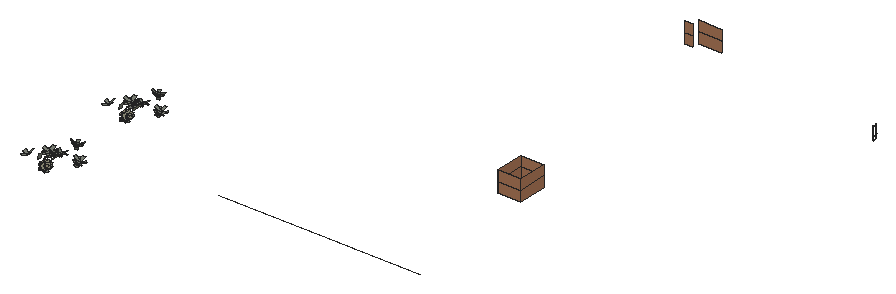
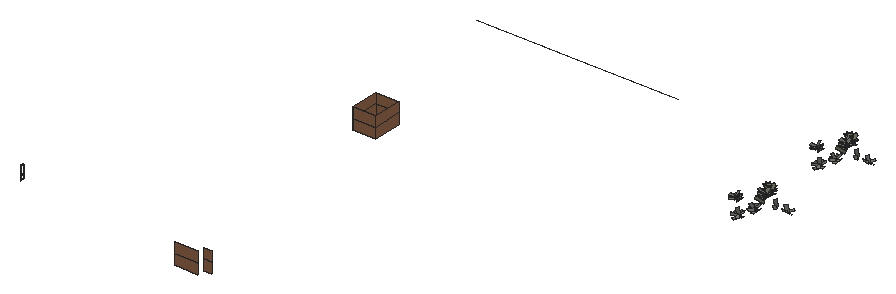
# SketchUp Ruby script. Lengths in inches.
U = 1.inch
M = Sketchup.active_model
def pt(a) = Geom::Point3d.new(a.map { |v| v * U })
def face(e, loops, mat)
  f = e.add_face(loops[0].map { |a| pt(a) })
  loops[1..].each { |l| e.add_face(l.map { |a| pt(a) }).erase! }
  f.material = f.back_material = mat if mat
  f
end
# faces: each face lists its corners as indices into pts; further lists are holes
def faces(e, pts, list, mat = nil) = list.each { |f| face(e, (f[0].is_a?(Array) ? f : [f]).map { |l| l.map { |i| pts[i] } }, mat) }
# xy, xz, yz: faces in a plane at the given z, y or x. An outline is a flat list of corners, or four numbers for a rectangle; further outlines are holes
def ring(l) = l.size == 4 ? [[l[0], l[1]], [l[2], l[1]], [l[2], l[3]], [l[0], l[3]]] : l.each_slice(2).to_a
def flat(e, list, mat, &to3) = list.each { |f| face(e, (f[0].is_a?(Array) ? f : [f]).map { |l| ring(l).map { |u, v| to3.(u, v) } }, mat) }
def xy(e, z, list, mat = nil) = flat(e, list, mat) { |x, y| [x, y, z] }
def xz(e, y, list, mat = nil) = flat(e, list, mat) { |x, z| [x, y, z] }
def yz(e, x, list, mat = nil) = flat(e, list, mat) { |y, z| [x, y, z] }
def lines(e, pts, list) = list.each { |a, b| e.add_line(pt(pts[a]), pt(pts[b])) }
# prism: a flat outline (further loops are holes) pulled along v
def prism(e, loops, v, mat = nil)
  f = face(e, loops, mat); d = Geom::Vector3d.new(v.map { |x| x * U })
  f.pushpull(f.normal.samedirection?(d) ? d.length : -d.length)
end
def box(e, o, s, mat = nil) = prism(e, [[o, [o[0] + s[0], o[1], o[2]], [o[0] + s[0], o[1] + s[1], o[2]], [o[0], o[1] + s[1], o[2]]]], [0, 0, s[2]], mat)
def at(x, y, z, deg = 0) = Geom::Transformation.translation(pt([x, y, z])) * Geom::Transformation.rotation(ORIGIN, Z_AXIS, deg.degrees)
def axes(o, x, y, z) = Geom::Transformation.new([*x, 0, *y, 0, *z, 0, *pt(o).to_a, 1])
def part(name) = M.definitions.add(name)
# library, detail: a bought-in or finely detailed component or shape, given as its bounding box
def library(name, o, s) = part(name).tap { |d| box(d.entities, o, s) }
def detail(e, o, s) = box(e.add_group.entities, o, s)
def put(e, d, t, mat = nil) = e.add_instance(d, t).tap { |i| i.material = mat if mat }
def group(e, t, mat = nil) = e.add_group.tap { |g| g.transformation = t; g.material = mat if mat }.entities
root = M.entities
M.materials.add("Material \#1").color = [140, 140, 140]
M.materials.add("[Tile Ceramic Multi]").color = [165, 115, 84]
M.materials.add("viburnumblaasdfas0df1w06d").color = [98, 102, 84]
M.materials.add("viburnumbladsadfasdfad0w122").color = [125, 129, 119]
M.materials.add("viburnumbloem1asdfas0d1fas0d616w").color = [137, 130, 109]
M.materials.add("viburnumbloem2asdfas01vxc5016").color = [175, 173, 148]
c1 = part("Component\#315")
p = [[0.25,0,0],[2.05,0.01,0.35],[1.81,4.2,1.66],[0,4.19,1.3125]]
faces(c1.entities,p,[[0,1,2,3]],"viburnumbladsadfasdfad0w122")
c2 = part("viburnumblad2")
put(c2.entities,c1,axes([-19.23,-4.49,-32.18],[83.35428,0,0],[0,79.38502,0],[0,0,83.35428]))
c3 = part("Component\#314")
p = [[0.14,0,0],[2.58,0.05,0.25],[2.44,5.11,2.64],[0,5.05,2.39]]
faces(c3.entities,p,[[0,1,2,3]],"viburnumblaasdfas0df1w06d")
c4 = part("viburnumblad1\#2")
put(c4.entities,c3,axes([-37.25,6.23,19.31],[75.98784,0,0],[0,65.50676,0],[0,0,75.98784]))
c5 = part("Component\#334")
p = [[0.16,3.84,5.17],[0,4.97,1.27],[3.78,1.125,0],[3.9375,0,3.9]]
faces(c5.entities,p,[[0,1,2,3]],"viburnumbloem2asdfas01vxc5016")
c6 = part("Component\#335")
p = [[1.35,5.21,5.35],[1.19,6.33,1.45],[0,1.125,0],[0.16,0,3.9]]
faces(c6.entities,p,[[0,1,2,3]],"viburnumbloem2asdfas01vxc5016")
c7 = part("Component\#333")
p = [[6.15,4.98,1.43],[0.18,5.1,1.71],[0,0.13,0.29],[5.97,0,0]]
faces(c7.entities,p,[[0,1,2,3]],"viburnumbloem1asdfas0d1fas0d616w")
c8 = part("Component\#336")
p = [[6.03,1.45,4.43],[5.85,2.68,0.17],[0,1.22,0],[0.18,0,4.25]]
faces(c8.entities,p,[[0,1,2,3]],"viburnumbloem2asdfas01vxc5016")
xz(root,340.216,[[1457.075,40,1474.638,48],[1457.075,48,1474.638,56]],"[Tile Ceramic Multi]")
xz(root,362.068,[[1457.075,40,1474.638,48],[1457.075,48,1474.638,56]],"[Tile Ceramic Multi]")
xz(root,529.3125,[[1590.723,42.477,1590.719,42.483,1590.583,42.689],[1590.719,42.483,1590.713,42.489,1590.583,42.689],[1590.713,42.489,1590.648,42.548,1590.583,42.689],[1590.713,42.489,1590.707,42.494,1590.648,42.548],[1590.707,42.494,1590.675,42.519,1590.648,42.548],
  [1590.648,42.548,1590.606,42.614,1590.583,42.689],[1590.648,42.548,1590.625,42.58,1590.606,42.614],[1590.686,42.562,1590.583,42.689,1590.651,42.612],[1590.651,42.612,1590.583,42.689,1590.628,42.668],[1590.606,42.614,1590.592,42.65,1590.583,42.689],
  [1590.628,42.668,1590.583,42.689,1590.62,42.729],[1590.583,42.689,1590.58,42.729,1590.589,42.798],[1590.583,42.689,1590.589,42.798,1590.655,42.918],[1590.583,42.689,1590.628,42.79,1590.62,42.729],[1590.583,42.689,1590.655,42.918,1590.628,42.79],
  [1590.628,42.79,1590.655,42.918,1590.651,42.846],[1590.589,42.798,1590.615,42.862,1590.655,42.918],[1590.651,42.846,1590.655,42.918,1590.686,42.896],[1590.686,42.896,1590.655,42.918,1590.733,42.9375],[1590.655,42.918,1590.708,42.965,1590.771,43.001],
  [1590.655,42.918,1590.788,42.969,1590.733,42.9375]],"Material \#1")
xz(root,529.347,[[1590.251,39.557,1590.17,39.659,1590.263,39.566],[1590.743,39.559,1590.698,39.58,1590.71,39.589],[1590.263,39.566,1590.17,39.659,1590.183,39.666],[1590.698,39.58,1590.669,39.616,1590.71,39.589],[1590.71,39.589,1590.669,39.616,1590.682,39.623],
  [1590.669,39.616,1590.648,39.657,1590.682,39.623],[1590.682,39.623,1590.648,39.657,1590.662,39.661],[1590.648,39.657,1590.634,39.701,1590.662,39.661],[1590.17,39.659,1590.1,39.787,1590.183,39.666],[1590.662,39.661,1590.634,39.701,1590.649,39.703],
  [1590.183,39.666,1590.1,39.787,1590.115,39.792],[1590.634,39.701,1590.63,39.742,1590.649,39.703],[1590.649,39.703,1590.63,39.742,1590.645,39.742],[1590.63,39.742,1590.634,39.793,1590.645,39.742],[1590.645,39.742,1590.634,39.793,1590.649,39.791],
  [1590.1,39.787,1590.06,39.918,1590.115,39.792],[1590.649,39.791,1590.634,39.793,1590.648,39.837],[1590.649,39.791,1590.648,39.837,1590.662,39.832],[1590.115,39.792,1590.06,39.918,1590.075,39.921],[1590.662,39.832,1590.648,39.837,1590.669,39.877],
  [1590.662,39.832,1590.669,39.877,1590.682,39.871],[1590.682,39.871,1590.669,39.877,1590.698,39.913],[1590.682,39.871,1590.698,39.913,1590.71,39.905],[1590.71,39.905,1590.698,39.913,1590.733,39.945],[1590.06,39.918,1590.045,40.063,1590.075,39.921],
  [1590.075,39.921,1590.045,40.063,1590.06,40.064],[1590.045,40.063,1590.045,48.955,1590.06,40.064],[1590.06,40.064,1590.045,48.955,1590.06,48.955],[1590.045,48.955,1590.06,49.1,1590.06,48.955],[1590.06,48.955,1590.06,49.1,1590.075,49.098],
  [1590.743,49.084,1590.698,49.105,1590.71,49.114],[1590.075,49.098,1590.06,49.1,1590.1,49.232],[1590.075,49.098,1590.1,49.232,1590.115,49.227],[1590.698,49.105,1590.669,49.141,1590.71,49.114],[1590.71,49.114,1590.669,49.141,1590.682,49.148],
  [1590.669,49.141,1590.648,49.182,1590.682,49.148],[1590.682,49.148,1590.648,49.182,1590.662,49.186],[1590.648,49.182,1590.634,49.226,1590.662,49.186],[1590.662,49.186,1590.634,49.226,1590.649,49.228],[1590.634,49.226,1590.63,49.284,1590.649,49.228],
  [1590.115,49.227,1590.1,49.232,1590.165,49.353],[1590.115,49.227,1590.165,49.353,1590.178,49.346],[1590.649,49.228,1590.63,49.284,1590.645,49.284],[1590.63,49.284,1590.634,49.318,1590.645,49.284],[1590.645,49.284,1590.634,49.318,1590.649,49.316],
  [1590.649,49.316,1590.634,49.318,1590.648,49.362],[1590.649,49.316,1590.648,49.362,1590.662,49.357],[1590.178,49.346,1590.165,49.353,1590.255,49.465],[1590.178,49.346,1590.255,49.465,1590.267,49.457],[1590.662,49.357,1590.648,49.362,1590.669,49.402],
  [1590.662,49.357,1590.669,49.402,1590.682,49.396],[1590.682,49.396,1590.669,49.402,1590.698,49.438],[1590.682,49.396,1590.698,49.438,1590.71,49.43],[1590.71,49.43,1590.698,49.438,1590.733,49.47],[1590.267,49.457,1590.255,49.465,1590.357,49.556],
  [1590.267,49.457,1590.357,49.556,1590.367,49.545],[1590.367,49.545,1590.357,49.556,1590.479,49.632],[1590.367,49.545,1590.479,49.632,1590.487,49.621],[1590.487,49.621,1590.479,49.632,1590.615,49.69],[1590.487,49.621,1590.615,49.69,1590.62,49.677],
  [1590.62,49.677,1590.615,49.69,1590.763,49.726],[1590.62,49.677,1590.763,49.726,1590.766,49.713]],"Material \#1")
xz(root,529.66,[[1590.723,42.477,1590.583,42.689,1590.719,42.483],[1590.723,42.477,1590.651,42.612,1590.583,42.689],[1590.723,42.477,1590.686,42.562,1590.651,42.612],[1590.719,42.483,1590.583,42.689,1590.713,42.489],[1590.713,42.489,1590.583,42.689,1590.648,42.548],
  [1590.713,42.489,1590.648,42.548,1590.707,42.494],[1590.707,42.494,1590.648,42.548,1590.675,42.519],[1590.648,42.548,1590.583,42.689,1590.606,42.614],[1590.648,42.548,1590.606,42.614,1590.625,42.58],[1590.651,42.612,1590.628,42.668,1590.583,42.689],
  [1590.606,42.614,1590.583,42.689,1590.592,42.65],[1590.628,42.668,1590.62,42.729,1590.583,42.689],[1590.583,42.689,1590.589,42.798,1590.58,42.729],[1590.583,42.689,1590.62,42.729,1590.628,42.79],[1590.583,42.689,1590.628,42.79,1590.651,42.846],
  [1590.583,42.689,1590.651,42.846,1590.655,42.918],[1590.583,42.689,1590.655,42.918,1590.589,42.798],[1590.589,42.798,1590.655,42.918,1590.615,42.862],[1590.651,42.846,1590.686,42.896,1590.655,42.918],[1590.686,42.896,1590.733,42.9375,1590.655,42.918],
  [1590.655,42.918,1590.771,43.001,1590.708,42.965]],"Material \#1")
xz(root,531.048,[[1590.723,42.477,1590.583,42.689,1590.651,42.612],[1590.723,42.477,1590.719,42.483,1590.583,42.689],[1590.723,42.477,1590.651,42.612,1590.686,42.562],[1590.719,42.483,1590.713,42.489,1590.583,42.689],[1590.713,42.489,1590.648,42.548,1590.583,42.689],
  [1590.713,42.489,1590.707,42.494,1590.648,42.548],[1590.707,42.494,1590.675,42.519,1590.648,42.548],[1590.648,42.548,1590.606,42.614,1590.583,42.689],[1590.648,42.548,1590.625,42.58,1590.606,42.614],[1590.651,42.612,1590.583,42.689,1590.628,42.668],
  [1590.606,42.614,1590.592,42.65,1590.583,42.689],[1590.628,42.668,1590.583,42.689,1590.62,42.729],[1590.583,42.689,1590.58,42.729,1590.589,42.798],[1590.583,42.689,1590.589,42.798,1590.655,42.918],[1590.583,42.689,1590.628,42.79,1590.62,42.729],
  [1590.583,42.689,1590.651,42.846,1590.628,42.79],[1590.583,42.689,1590.655,42.918,1590.651,42.846],[1590.589,42.798,1590.615,42.862,1590.655,42.918],[1590.651,42.846,1590.655,42.918,1590.686,42.896],[1590.686,42.896,1590.655,42.918,1590.733,42.9375],
  [1590.655,42.918,1590.708,42.965,1590.771,43.001]],"Material \#1")
xz(root,531.361,[[1590.251,39.557,1590.263,39.566,1590.17,39.659],[1590.263,39.566,1590.183,39.666,1590.17,39.659],[1590.698,39.58,1590.71,39.589,1590.669,39.616],[1590.71,39.589,1590.682,39.623,1590.669,39.616],[1590.669,39.616,1590.682,39.623,1590.648,39.657],
  [1590.682,39.623,1590.662,39.661,1590.648,39.657],[1590.648,39.657,1590.662,39.661,1590.634,39.701],[1590.17,39.659,1590.183,39.666,1590.1,39.787],[1590.662,39.661,1590.649,39.703,1590.634,39.701],[1590.183,39.666,1590.115,39.792,1590.1,39.787],
  [1590.634,39.701,1590.649,39.703,1590.63,39.742],[1590.649,39.703,1590.645,39.742,1590.63,39.742],[1590.63,39.742,1590.645,39.742,1590.634,39.793],[1590.645,39.742,1590.649,39.791,1590.634,39.793],[1590.1,39.787,1590.115,39.792,1590.06,39.918],
  [1590.649,39.791,1590.648,39.837,1590.634,39.793],[1590.649,39.791,1590.662,39.832,1590.648,39.837],[1590.115,39.792,1590.075,39.921,1590.06,39.918],[1590.662,39.832,1590.669,39.877,1590.648,39.837],[1590.662,39.832,1590.682,39.871,1590.669,39.877],
  [1590.682,39.871,1590.698,39.913,1590.669,39.877],[1590.682,39.871,1590.71,39.905,1590.698,39.913],[1590.71,39.905,1590.733,39.945,1590.698,39.913],[1590.06,39.918,1590.075,39.921,1590.045,40.063],[1590.075,39.921,1590.06,40.064,1590.045,40.063],
  [1590.045,40.063,1590.06,40.064,1590.045,48.955],[1590.06,40.064,1590.06,48.955,1590.045,48.955],[1590.045,48.955,1590.06,48.955,1590.06,49.1],[1590.06,48.955,1590.075,49.098,1590.06,49.1],[1590.075,49.098,1590.1,49.232,1590.06,49.1],
  [1590.075,49.098,1590.115,49.227,1590.1,49.232],[1590.698,49.105,1590.71,49.114,1590.669,49.141],[1590.71,49.114,1590.682,49.148,1590.669,49.141],[1590.669,49.141,1590.682,49.148,1590.648,49.182],[1590.682,49.148,1590.662,49.186,1590.648,49.182],
  [1590.648,49.182,1590.662,49.186,1590.634,49.226],[1590.662,49.186,1590.649,49.228,1590.634,49.226],[1590.634,49.226,1590.649,49.228,1590.63,49.284],[1590.115,49.227,1590.165,49.353,1590.1,49.232],[1590.115,49.227,1590.178,49.346,1590.165,49.353],
  [1590.649,49.228,1590.645,49.284,1590.63,49.284],[1590.63,49.284,1590.645,49.284,1590.634,49.318],[1590.645,49.284,1590.649,49.316,1590.634,49.318],[1590.649,49.316,1590.648,49.362,1590.634,49.318],[1590.649,49.316,1590.662,49.357,1590.648,49.362],
  [1590.178,49.346,1590.255,49.465,1590.165,49.353],[1590.178,49.346,1590.267,49.457,1590.255,49.465],[1590.662,49.357,1590.669,49.402,1590.648,49.362],[1590.662,49.357,1590.682,49.396,1590.669,49.402],[1590.682,49.396,1590.698,49.438,1590.669,49.402],
  [1590.682,49.396,1590.71,49.43,1590.698,49.438],[1590.71,49.43,1590.733,49.47,1590.698,49.438],[1590.267,49.457,1590.357,49.556,1590.255,49.465],[1590.267,49.457,1590.367,49.545,1590.357,49.556],[1590.367,49.545,1590.479,49.632,1590.357,49.556],
  [1590.367,49.545,1590.487,49.621,1590.479,49.632],[1590.487,49.621,1590.615,49.69,1590.479,49.632],[1590.487,49.621,1590.62,49.677,1590.615,49.69],[1590.62,49.677,1590.763,49.726,1590.615,49.69],[1590.62,49.677,1590.766,49.713,1590.763,49.726]],"Material \#1")
xz(root,531.396,[[1590.723,42.477,1590.583,42.689,1590.719,42.483],[1590.719,42.483,1590.583,42.689,1590.713,42.489],[1590.713,42.489,1590.583,42.689,1590.648,42.548],[1590.713,42.489,1590.648,42.548,1590.707,42.494],[1590.707,42.494,1590.648,42.548,1590.675,42.519],
  [1590.648,42.548,1590.583,42.689,1590.606,42.614],[1590.648,42.548,1590.606,42.614,1590.625,42.58],[1590.686,42.562,1590.651,42.612,1590.583,42.689],[1590.651,42.612,1590.628,42.668,1590.583,42.689],[1590.606,42.614,1590.583,42.689,1590.592,42.65],
  [1590.628,42.668,1590.62,42.729,1590.583,42.689],[1590.583,42.689,1590.589,42.798,1590.58,42.729],[1590.583,42.689,1590.62,42.729,1590.628,42.79],[1590.583,42.689,1590.628,42.79,1590.655,42.918],[1590.583,42.689,1590.655,42.918,1590.589,42.798],
  [1590.628,42.79,1590.651,42.846,1590.655,42.918],[1590.589,42.798,1590.655,42.918,1590.615,42.862],[1590.651,42.846,1590.686,42.896,1590.655,42.918],[1590.686,42.896,1590.733,42.9375,1590.655,42.918],[1590.655,42.918,1590.771,43.001,1590.708,42.965]],"Material \#1")
xz(root,549.6875,[[1431.3125,40,1437.219,48],[1431.3125,48,1437.219,56]],"[Tile Ceramic Multi]")
xz(root,555,[[1437.219,40,1454.9375,48],[1437.219,48,1454.9375,56]],"[Tile Ceramic Multi]")
yz(root,1457.075,[[340.216,40,362.068,48],[340.216,48,362.068,56]],"[Tile Ceramic Multi]")
yz(root,1474.638,[[340.216,40,362.068,48],[340.216,48,362.068,56]],"[Tile Ceramic Multi]")
p = [[1491.419,223.9375,48],[1338.625,223.9375,48]]
lines(root,p,[[0,1]])
put(root,c2,axes([1210.86,278.68,40.57],[0.00639,0.01034,0.00318],[-0.01046,0.00683,-0.00122],[-0.00247,-0.00201,0.01151]))
put(root,c2,axes([1210.86,201.8,40.57],[0.00639,0.01034,0.00318],[-0.01046,0.00683,-0.00122],[-0.00247,-0.00201,0.01151]))
put(root,c2,axes([1212.37,278.7,41.07],[-0.01008,0.00703,-0.00261],[-0.00679,-0.01041,-0.00178],[-0.00292,0.0001,0.01158]))
put(root,c2,axes([1212.37,201.82,41.07],[-0.01008,0.00703,-0.00261],[-0.00679,-0.01041,-0.00178],[-0.00292,0.0001,0.01158]))
put(root,c2,axes([1210.79,280.26,40.71],[0.01008,-0.00703,0.00261],[0.00588,0.01012,0.00453],[-0.00448,-0.00242,0.01081]))
put(root,c2,axes([1210.79,203.375,40.71],[0.01008,-0.00703,0.00261],[0.00588,0.01012,0.00453],[-0.00448,-0.00242,0.01081]))
put(root,c2,axes([1212.29,280.28,41.21],[-0.00639,-0.01034,-0.00318],[0.00955,-0.00712,0.00396],[-0.00493,-0.0003,0.01087]))
put(root,c2,axes([1212.29,203.4,41.21],[-0.00639,-0.01034,-0.00318],[0.00955,-0.00712,0.00396],[-0.00493,-0.0003,0.01087]))
put(root,c2,axes([1218.84,279.94,40.32],[0.00996,-0.00362,0.00815],[0.00104,0.0126,0.00432],[-0.00886,-0.00258,0.00967]))
put(root,c2,axes([1218.84,203.0625,40.32],[0.00996,-0.00362,0.00815],[0.00104,0.0126,0.00432],[-0.00886,-0.00258,0.00967]))
put(root,c2,axes([1220.02,280.5,41.38],[-0.00212,-0.01282,-0.00311],[0.00883,-0.00372,0.00932],[-0.00981,-0.00058,0.00906]))
put(root,c2,axes([1220.02,203.62,41.38],[-0.00212,-0.01282,-0.00311],[0.00883,-0.00372,0.00932],[-0.00981,-0.00058,0.00906]))
put(root,c2,axes([1227.75,278.98,47.84],[0,0.0133,0.00135],[-0.01327,-0.00016,0.00162],[0.00163,-0.00134,0.0132]))
put(root,c2,axes([1227.75,202.1,47.84],[0,0.0133,0.00135],[-0.01327,-0.00016,0.00162],[0.00163,-0.00134,0.0132]))
put(root,c2,axes([1227.03,289.83,42.27],[0.00628,0.01038,-0.00277],[-0.0108,0.0064,-0.00025],[0.00133,0.00298,0.0111]))
put(root,c2,axes([1227.03,212.95,42.27],[0.00628,0.01038,-0.00277],[-0.0108,0.0064,-0.00025],[0.00133,0.00298,0.0111]))
put(root,c2,axes([1228.03,289.1,40.9],[-0.00325,0.01157,-0.00309],[-0.01106,-0.00241,0.00198],[0.00148,0.00409,0.01081]))
put(root,c2,axes([1228.03,212.22,40.9],[-0.00325,0.01157,-0.00309],[-0.01106,-0.00241,0.00198],[0.00148,0.00409,0.01081]))
put(root,c2,axes([1227.13,279.55,46.2],[0.00945,0.0094,0.00096],[-0.00938,0.00917,0.00257],[0.00115,-0.00249,0.01308]))
put(root,c2,axes([1227.13,202.67,46.2],[0.00945,0.0094,0.00096],[-0.00938,0.00917,0.00257],[0.00115,-0.00249,0.01308]))
put(root,c2,axes([1228.83,279.29,46.17],[-0.00945,0.0094,0.00096],[-0.00947,-0.00959,0.00068],[0.00115,-0.00019,0.01331]))
put(root,c2,axes([1228.83,202.41,46.17],[-0.00945,0.0094,0.00096],[-0.00947,-0.00959,0.00068],[0.00115,-0.00019,0.01331]))
put(root,c2,axes([1226.5,289.96,40.71],[0.01214,0.0031,-0.00083],[-0.00326,0.01206,-0.00174],[0.0004,0.0023,0.01128]))
put(root,c2,axes([1226.5,213.08,40.71],[0.01214,0.0031,-0.00083],[-0.00326,0.01206,-0.00174],[0.0004,0.0023,0.01128]))
put(root,c2,axes([1228.61,289.97,42.23],[-0.01088,0.00599,-0.0016],[-0.00623,-0.00984,0.00409],[0.00077,0.00497,0.01057]))
put(root,c2,axes([1228.61,213.08,42.23],[-0.01088,0.00599,-0.0016],[-0.00623,-0.00984,0.00409],[0.00077,0.00497,0.01057]))
put(root,c2,axes([1229.21,302.375,42.25],[0.00325,0.01134,-0.00432],[-0.01209,0.00342,-0.00014],[0.00105,0.00419,0.0118]))
put(root,c2,axes([1229.21,225.49,42.25],[0.00325,0.01134,-0.00432],[-0.01209,0.00342,-0.00014],[0.00105,0.00419,0.0118]))
put(root,c2,axes([1226.78,280.35,47.98],[0.01337,0,0],[0,0.01303,0.00296],[0,-0.00296,0.01303]))
put(root,c2,axes([1226.78,203.47,47.98],[0.01337,0,0],[0,0.01303,0.00296],[0,-0.00296,0.01303]))
put(root,c2,axes([1229.85,302.93,43.77],[-0.00627,0.01006,-0.00416],[-0.01085,-0.00538,0.00335],[0.0009,0.00527,0.01137]))
put(root,c2,axes([1229.85,226.05,43.77],[-0.00627,0.01006,-0.00416],[-0.01085,-0.00538,0.00335],[0.0009,0.00527,0.01137]))
put(root,c2,axes([1227.0625,280.39,44.625],[0.01283,0,0],[0,0.01408,0.0032],[0,-0.00296,0.01303]))
put(root,c2,axes([1227.0625,203.51,44.625],[0.01283,0,0],[0,0.01408,0.0032],[0,-0.00296,0.01303]))
put(root,c2,axes([1228.41,303.53,43.48],[0.01088,0.00598,-0.00194],[-0.00628,0.01054,-0.00271],[0.00034,0.00331,0.01211]))
put(root,c2,axes([1228.41,226.65,43.48],[0.01088,0.00598,-0.00194],[-0.00628,0.01054,-0.00271],[0.00034,0.00331,0.01211]))
put(root,c2,axes([1229.13,279.95,47.94],[-0.01337,0,0],[0,-0.01336,0.00028],[0,0.00028,0.01336]))
put(root,c2,axes([1229.13,203.06,47.94],[-0.01337,0,0],[0,-0.01336,0.00028],[0,0.00028,0.01336]))
put(root,c2,axes([1229.25,280.34,44.77],[-0.01222,-0.00003,-0.00133],[0,-0.01336,0.00028],[-0.00144,0.00028,0.01328]))
put(root,c2,axes([1229.25,203.46,44.77],[-0.01222,-0.00003,-0.00133],[0,-0.01336,0.00028],[-0.00144,0.00028,0.01328]))
put(root,c2,axes([1228.67,290.38,40.57],[-0.01214,-0.0031,0.00083],[0.00339,-0.01158,0.00463],[-0.0004,0.00512,0.01053]))
put(root,c2,axes([1228.67,213.5,40.57],[-0.01214,-0.0031,0.00083],[0.00339,-0.01158,0.00463],[-0.0004,0.00512,0.01053]))
put(root,c2,axes([1226.89,291.34,41.86],[0.01088,-0.00599,0.0016],[0.00623,0.01076,-0.00141],[-0.00077,0.00244,0.01124]))
put(root,c2,axes([1226.89,214.46,41.86],[0.01088,-0.00599,0.0016],[0.00623,0.01076,-0.00141],[-0.00077,0.00244,0.01124]))
put(root,c2,axes([1230.71,302.9375,42.08],[-0.01213,0.00288,-0.00157],[-0.00331,-0.01081,0.00577],[-0.00003,0.00592,0.01108]))
put(root,c2,axes([1230.71,226.06,42.08],[-0.01213,0.00288,-0.00157],[-0.00331,-0.01081,0.00577],[-0.00003,0.00592,0.01108]))
put(root,c2,axes([1227.26,281.05,46.32],[0.00945,-0.0094,-0.00096],[0.00985,0.00963,0.0027],[-0.00115,-0.00249,0.01308]))
put(root,c2,axes([1227.26,204.17,46.32],[0.00945,-0.0094,-0.00096],[0.00985,0.00963,0.0027],[-0.00115,-0.00249,0.01308]))
put(root,c2,axes([1228.83,281.17,46.32],[-0.00945,-0.0094,-0.00096],[0.00861,-0.00872,0.00062],[-0.00115,-0.00019,0.01331]))
put(root,c2,axes([1228.83,204.29,46.32],[-0.00945,-0.0094,-0.00096],[0.00861,-0.00872,0.00062],[-0.00115,-0.00019,0.01331]))
put(root,c2,axes([1227.5,291.16,40.39],[0.00325,-0.01157,0.00309],[0.01204,0.00353,0.00052],[-0.00148,0.00333,0.01101]))
put(root,c2,axes([1227.5,214.28,40.39],[0.00325,-0.01157,0.00309],[0.01204,0.00353,0.00052],[-0.00148,0.00333,0.01101]))
put(root,c2,axes([1228.47,291.47,41.83],[-0.00628,-0.01038,0.00277],[0.0108,-0.00549,0.00293],[-0.00133,0.00444,0.01071]))
put(root,c2,axes([1228.47,214.59,41.83],[-0.00628,-0.01038,0.00277],[0.0108,-0.00549,0.00293],[-0.00133,0.00444,0.01071]))
put(root,c2,axes([1228.61,303.55,41.74],[0.01213,-0.00288,0.00157],[0.00334,0.0124,-0.003],[-0.00082,0.00316,0.01213]))
put(root,c2,axes([1228.61,226.67,41.74],[0.01213,-0.00288,0.00157],[0.00334,0.0124,-0.003],[-0.00082,0.00316,0.01213]))
put(root,c4,axes([1227.69,281.85,41.43],[0.00718,-0.01267,0.00168],[0.01433,0.00855,0.00326],[-0.00327,0.00004,0.01429]))
put(root,c4,axes([1227.69,204.97,41.43],[0.00718,-0.01267,0.00168],[0.01433,0.00855,0.00326],[-0.00327,0.00004,0.01429]))
put(root,c2,axes([1228.36,281.48,44.78],[0,-0.01388,-0.00141],[0.01194,-0.00015,0.00146],[-0.00163,-0.00134,0.0132]))
put(root,c2,axes([1228.36,204.6,44.78],[0,-0.01388,-0.00141],[0.01194,-0.00015,0.00146],[-0.00163,-0.00134,0.0132]))
put(root,c2,axes([1228.16,281.32,48.08],[0,-0.0133,-0.00135],[0.01327,-0.00016,0.00162],[-0.00163,-0.00134,0.0132]))
put(root,c2,axes([1228.16,204.4375,48.08],[0,-0.0133,-0.00135],[0.01327,-0.00016,0.00162],[-0.00163,-0.00134,0.0132]))
put(root,c2,axes([1230.51,304.28,43.27],[-0.01088,-0.00598,0.00194],[0.00618,-0.00942,0.00556],[-0.00119,0.00576,0.0111]))
put(root,c2,axes([1230.51,227.4,43.27],[-0.01088,-0.00598,0.00194],[0.00618,-0.00942,0.00556],[-0.00119,0.00576,0.0111]))
put(root,c2,axes([1232.55,269.29,40.37],[0.00044,0.0126,0.00361],[-0.01115,-0.00014,0.00186],[0.00203,-0.00348,0.0119]))
put(root,c2,axes([1232.55,192.4,40.37],[0.00044,0.0126,0.00361],[-0.01115,-0.00014,0.00186],[0.00203,-0.00348,0.0119]))
put(root,c2,axes([1230.68,303.29,40.43],[-0.00983,-0.00604,0.00067],[0.00618,-0.00942,0.00556],[-0.00236,0.00509,0.01124]))
put(root,c2,axes([1230.68,226.41,40.43],[-0.00983,-0.00604,0.00067],[0.00618,-0.00942,0.00556],[-0.00236,0.00509,0.01124]))
put(root,c2,axes([1232.86,268.26,43.3],[0.00042,0.01207,0.00346],[-0.01239,-0.00016,0.00207],[0.00203,-0.00348,0.0119]))
put(root,c2,axes([1232.86,191.38,43.3],[0.00042,0.01207,0.00346],[-0.01239,-0.00016,0.00207],[0.00203,-0.00348,0.0119]))
put(root,c2,axes([1229.07,304.88,42.98],[0.00627,-0.01006,0.00416],[0.01074,0.0065,-0.0005],[-0.00175,0.00381,0.01184]))
put(root,c2,axes([1229.07,228,42.98],[0.00627,-0.01006,0.00416],[0.01074,0.0065,-0.0005],[-0.00175,0.00381,0.01184]))
put(root,c2,axes([1229.83,304.34,41.46],[-0.00325,-0.01134,0.00432],[0.011,-0.00211,0.00274],[-0.0019,0.00489,0.01141]))
put(root,c2,axes([1229.83,227.46,41.46],[-0.00325,-0.01134,0.00432],[0.011,-0.00211,0.00274],[-0.0019,0.00489,0.01141]))
put(root,c2,axes([1232.17,269.02,41.84],[0.00917,0.00834,0.00202],[-0.00775,0.00756,0.00397],[0.00155,-0.00451,0.01162]))
put(root,c2,axes([1232.17,192.14,41.84],[0.00917,0.00834,0.00202],[-0.00775,0.00756,0.00397],[0.00155,-0.00451,0.01162]))
put(root,c2,axes([1233.65,269.1,41.82],[-0.00857,0.00873,0.00287],[-0.00949,-0.00914,-0.00056],[0.00162,-0.00243,0.01222]))
put(root,c2,axes([1233.65,192.22,41.82],[-0.00857,0.00873,0.00287],[-0.00949,-0.00914,-0.00056],[0.00162,-0.00243,0.01222]))
put(root,c2,axes([1231.76,270.3,40.8],[0.01143,0.00024,-0.0017],[0.00048,0.01156,0.0049],[0.0018,-0.00492,0.01142]))
put(root,c2,axes([1231.76,193.42,40.8],[0.01143,0.00024,-0.0017],[0.00048,0.01156,0.0049],[0.0018,-0.00492,0.01142]))
put(root,c2,axes([1231.99,269.53,43.7],[0.01255,-0.00027,-0.0006],[0.00048,0.01156,0.0049],[0.00045,-0.00492,0.01155]))
put(root,c2,axes([1231.99,192.65,43.7],[0.01255,-0.00027,-0.0006],[0.00048,0.01156,0.0049],[0.00045,-0.00492,0.01155]))
put(root,c5,axes([1231.11,266.3,42.93],[1.0472,0,0],[0,1.0472,0],[0,0,1.0472]))
put(root,c5,axes([1231.11,189.41,42.93],[1.0472,0,0],[0,1.0472,0],[0,0,1.0472]))
put(root,c2,axes([1234.18,269.11,43.49],[-0.01255,0.00027,0.0006],[-0.00036,-0.0124,-0.00196],[0.00055,-0.00198,0.01239]))
put(root,c2,axes([1234.18,192.23,43.49],[-0.01255,0.00027,0.0006],[-0.00036,-0.0124,-0.00196],[0.00055,-0.00198,0.01239]))
put(root,c6,axes([1232.62,265.67,42.85],[1.0472,0,0],[0,1.0472,0],[0,0,1.0472]))
put(root,c6,axes([1232.62,188.78,42.85],[1.0472,0,0],[0,1.0472,0],[0,0,1.0472]))
put(root,c7,axes([1230.11,266.375,45.82],[1.0472,0,0],[0,1.0472,0],[0,0,1.0472]))
put(root,c7,axes([1230.11,189.49,45.82],[1.0472,0,0],[0,1.0472,0],[0,0,1.0472]))
put(root,c8,axes([1230.36,267.44,43.24],[1.0472,0,0],[0,1.0472,0],[0,0,1.0472]))
put(root,c8,axes([1230.36,190.5625,43.24],[1.0472,0,0],[0,1.0472,0],[0,0,1.0472]))
put(root,c2,axes([1232.24,270.72,42.36],[0.00857,-0.00873,-0.00287],[0.00926,0.00794,0.00351],[-0.00062,-0.00447,0.01173]))
put(root,c2,axes([1232.24,193.83,42.36],[0.00857,-0.00873,-0.00287],[0.00926,0.00794,0.00351],[-0.00062,-0.00447,0.01173]))
put(root,c2,axes([1233.82,270.45,42.23],[-0.00917,-0.00834,-0.00202],[0.00857,-0.00908,-0.00138],[-0.00054,-0.00239,0.01232]))
put(root,c2,axes([1233.82,193.57,42.23],[-0.00917,-0.00834,-0.00202],[0.00857,-0.00908,-0.00138],[-0.00054,-0.00239,0.01232]))
put(root,c2,axes([1233.32,270.38,43.89],[-0.00042,-0.01207,-0.00346],[0.01251,-0.00069,0.00087],[-0.00103,-0.00342,0.01205]))
put(root,c2,axes([1233.32,193.5,43.89],[-0.00042,-0.01207,-0.00346],[0.01251,-0.00069,0.00087],[-0.00103,-0.00342,0.01205]))
put(root,c2,axes([1243.12,286.625,40.8],[-0.00024,0.01143,-0.0017],[-0.01156,0.00048,0.0049],[0.00492,0.0018,0.01142]))
put(root,c2,axes([1243.12,209.74,40.8],[-0.00024,0.01143,-0.0017],[-0.01156,0.00048,0.0049],[0.00492,0.0018,0.01142]))
put(root,c2,axes([1242.71,287.1,42.36],[0.00873,0.00857,-0.00287],[-0.00794,0.00926,0.00351],[0.00447,-0.00062,0.01173]))
put(root,c2,axes([1242.71,210.22,42.36],[0.00873,0.00857,-0.00287],[-0.00794,0.00926,0.00351],[0.00447,-0.00062,0.01173]))
put(root,c2,axes([1243.89,286.85,43.7],[0.00027,0.01255,-0.0006],[-0.01156,0.00048,0.0049],[0.00492,0.00045,0.01155]))
put(root,c2,axes([1243.89,209.97,43.7],[0.00027,0.01255,-0.0006],[-0.01156,0.00048,0.0049],[0.00492,0.00045,0.01155]))
put(root,c2,axes([1244.4,287.04,41.84],[-0.00834,0.00917,0.00202],[-0.00756,-0.00775,0.00397],[0.00451,0.00155,0.01162]))
put(root,c2,axes([1244.4,210.16,41.84],[-0.00834,0.00917,0.00202],[-0.00756,-0.00775,0.00397],[0.00451,0.00155,0.01162]))
put(root,c2,axes([1244.14,287.42,40.37],[-0.0126,0.00044,0.00361],[0.00014,-0.01115,0.00186],[0.00348,0.00203,0.0119]))
put(root,c2,axes([1244.14,210.53,40.37],[-0.0126,0.00044,0.00361],[0.00014,-0.01115,0.00186],[0.00348,0.00203,0.0119]))
put(root,c2,axes([1243.04,288.18,43.89],[0.01207,-0.00042,-0.00346],[0.00069,0.01251,0.00087],[0.00342,-0.00103,0.01205]))
put(root,c2,axes([1243.04,211.3,43.89],[0.01207,-0.00042,-0.00346],[0.00069,0.01251,0.00087],[0.00342,-0.00103,0.01205]))
put(root,c2,axes([1245.16,287.72,43.3],[-0.01207,0.00042,0.00346],[0.00016,-0.01239,0.00207],[0.00348,0.00203,0.0119]))
put(root,c2,axes([1245.16,210.84,43.3],[-0.01207,0.00042,0.00346],[0.00016,-0.01239,0.00207],[0.00348,0.00203,0.0119]))
put(root,c2,axes([1242.98,288.68,42.23],[0.00834,-0.00917,-0.00202],[0.00908,0.00857,-0.00138],[0.00239,-0.00054,0.01232]))
put(root,c2,axes([1242.98,211.8,42.23],[0.00834,-0.00917,-0.00202],[0.00908,0.00857,-0.00138],[0.00239,-0.00054,0.01232]))
put(root,c2,axes([1244.32,288.51,41.82],[-0.00873,-0.00857,0.00287],[0.00914,-0.00949,-0.00056],[0.00243,0.00162,0.01222]))
put(root,c2,axes([1244.32,211.63,41.82],[-0.00873,-0.00857,0.00287],[0.00914,-0.00949,-0.00056],[0.00243,0.00162,0.01222]))
put(root,c2,axes([1244.31,289.05,43.49],[-0.00027,-0.01255,0.0006],[0.0124,-0.00036,-0.00196],[0.00198,0.00055,0.01239]))
put(root,c2,axes([1244.31,212.17,43.49],[-0.00027,-0.01255,0.0006],[0.0124,-0.00036,-0.00196],[0.00198,0.00055,0.01239]))
